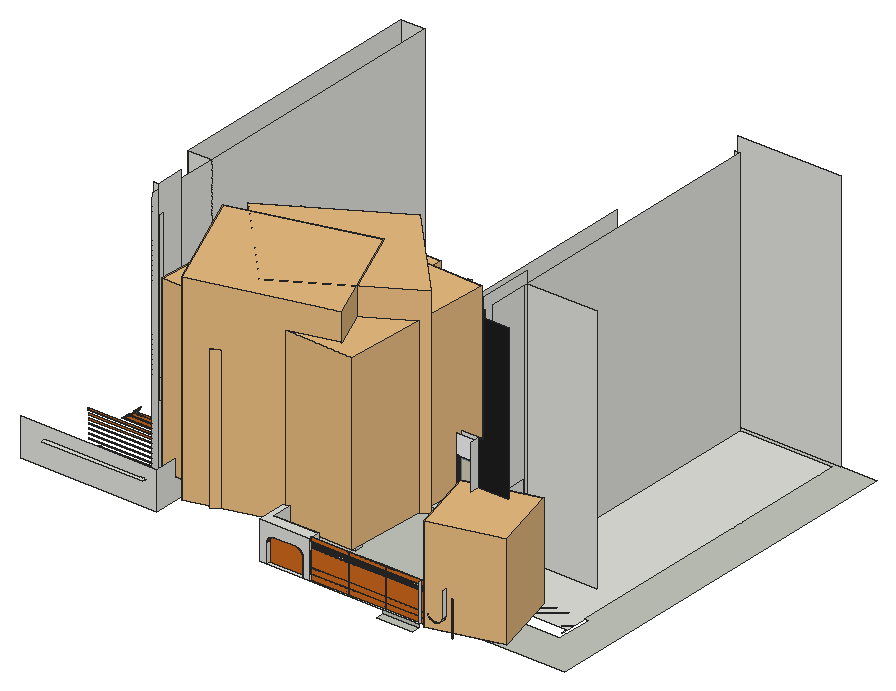
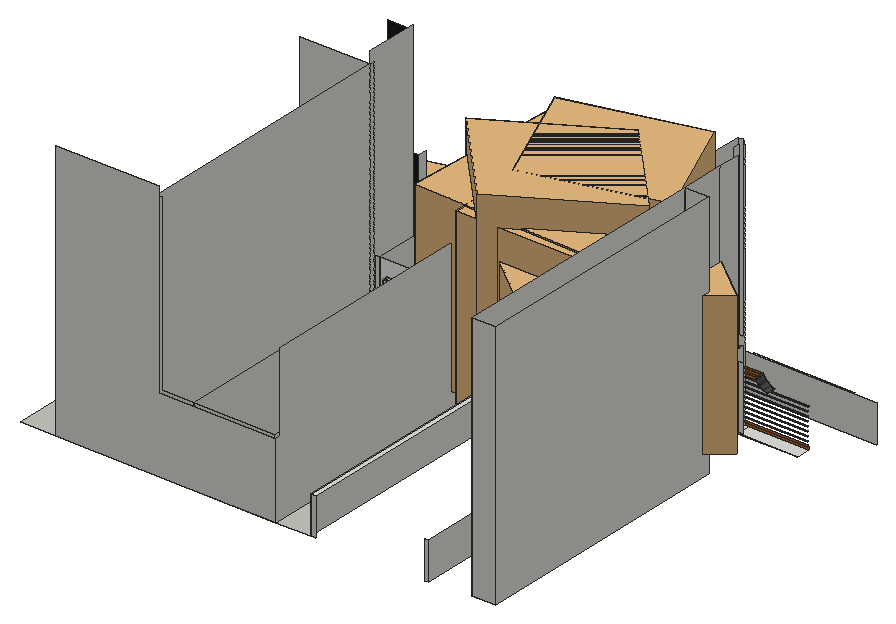
# SketchUp Ruby script. Lengths in inches.
U = 1.inch
M = Sketchup.active_model
def pt(a) = Geom::Point3d.new(a.map { |v| v * U })
def face(e, loops, mat)
  f = e.add_face(loops[0].map { |a| pt(a) })
  loops[1..].each { |l| e.add_face(l.map { |a| pt(a) }).erase! }
  f.material = f.back_material = mat if mat
  f
end
# faces: each face lists its corners as indices into pts; further lists are holes
def faces(e, pts, list, mat = nil) = list.each { |f| face(e, (f[0].is_a?(Array) ? f : [f]).map { |l| l.map { |i| pts[i] } }, mat) }
# xy, xz, yz: faces in a plane at the given z, y or x. An outline is a flat list of corners, or four numbers for a rectangle; further outlines are holes
def ring(l) = l.size == 4 ? [[l[0], l[1]], [l[2], l[1]], [l[2], l[3]], [l[0], l[3]]] : l.each_slice(2).to_a
def flat(e, list, mat, &to3) = list.each { |f| face(e, (f[0].is_a?(Array) ? f : [f]).map { |l| ring(l).map { |u, v| to3.(u, v) } }, mat) }
def xy(e, z, list, mat = nil) = flat(e, list, mat) { |x, y| [x, y, z] }
def xz(e, y, list, mat = nil) = flat(e, list, mat) { |x, z| [x, y, z] }
def yz(e, x, list, mat = nil) = flat(e, list, mat) { |y, z| [x, y, z] }
def lines(e, pts, list) = list.each { |a, b| e.add_line(pt(pts[a]), pt(pts[b])) }
# prism: a flat outline (further loops are holes) pulled along v
def prism(e, loops, v, mat = nil)
  f = face(e, loops, mat); d = Geom::Vector3d.new(v.map { |x| x * U })
  f.pushpull(f.normal.samedirection?(d) ? d.length : -d.length)
end
def box(e, o, s, mat = nil) = prism(e, [[o, [o[0] + s[0], o[1], o[2]], [o[0] + s[0], o[1] + s[1], o[2]], [o[0], o[1] + s[1], o[2]]]], [0, 0, s[2]], mat)
def at(x, y, z, deg = 0) = Geom::Transformation.translation(pt([x, y, z])) * Geom::Transformation.rotation(ORIGIN, Z_AXIS, deg.degrees)
def axes(o, x, y, z) = Geom::Transformation.new([*x, 0, *y, 0, *z, 0, *pt(o).to_a, 1])
def part(name) = M.definitions.add(name)
# library, detail: a bought-in or finely detailed component or shape, given as its bounding box
def library(name, o, s) = part(name).tap { |d| box(d.entities, o, s) }
def detail(e, o, s) = box(e.add_group.entities, o, s)
def put(e, d, t, mat = nil) = e.add_instance(d, t).tap { |i| i.material = mat if mat }
def group(e, t, mat = nil) = e.add_group.tap { |g| g.transformation = t; g.material = mat if mat }.entities
root = M.entities
M.materials.add("[0041_Chocolate]").color = [210, 105, 30]
M.materials.add("[0129_WhiteSmoke]").color = [245, 245, 245]
M.materials.add("[Color M06]").color = [84, 84, 84]
M.materials.add("[Color M08]").color = [30, 30, 30]
M.materials.add("[Pavers with Grass Herringbone]").color = [197, 201, 190]
M.materials.add("[Translucent Glass Safety]").color = [204, 235, 244]
M.materials["[Translucent Glass Safety]"].alpha = 0.5
M.materials.add("[Wood Veneer 01]").color = [120, 70, 37]
M.materials.add("[Wood Veneer 01]2").color = [94, 55, 29]
c1 = library("Group\#287",[-33.32,-34.9375,32.67],[162.87,159.66,128.34])
c2 = library("Group\#288",[-10.45,-6.67,0],[121.7,116.61,164.95])
c3 = library("Group\#286",[-10.45,-6.67,0],[121.7,116.61,164.95])
c4 = library("Group\#284",[-10.45,-6.67,0],[121.7,116.61,164.95])
c5 = library("Group\#283",[-33.32,-34.9375,32.67],[162.87,159.66,128.34])
c6 = library("Group\#285",[-33.32,-34.9375,81.35],[162.87,159.66,79.66])
c7 = library("Group\#282",[-33.32,-34.9375,77.91],[162.87,159.66,83.1])
c8 = part("Palem Elek")
put(c8.entities,c1,axes([92.2,20.3,-29.73],[0.70711,0.70711,0],[-0.70711,0.70711,0],[0,0,0.91208]))
put(c8.entities,c2,axes([60.27,20.78,0],[1,0,0],[0,1,0],[0,0,0.85762]))
put(c8.entities,c3,at(25.45,60.83,0,-53.5))
put(c8.entities,c4,at(84.4375,135.48,0,-161.4))
put(c8.entities,c5,axes([38.54,105.7,-36.19],[-0.04013,-0.99919,0],[0.99919,-0.04013,0],[0,0,1.11001]))
put(c8.entities,c6,axes([57.15,96.51,-54.45],[-0.02003,-0.49872,0.02965],[0.4996,-0.02007,0],[0.00123,0.03065,0.51628]))
put(c8.entities,c7,axes([74.94,50.39,-54.06],[0.40095,0.29715,0.03075],[-0.29654,0.38966,0.10114],[0.04012,-0.11026,0.54246]))
c9 = part("palem elek\#1")
put(c9.entities,c8,at(-81.14,-74.56,-0.83))
c10 = part("Coqueiro")
put(c10.entities,c9,axes([83.17,89.39,9.5625],[0,1.1016,0],[-1.377,0,0],[0,0,1.39284]))
c11 = part("Slatted screen panel")
xy(c11.entities,0,[[0,0,255.91,1.97]],"[Wood Veneer 01]2")
xy(c11.entities,16.54,[[0,1.18,255.91,1.97]],"[Wood Veneer 01]2")
xy(c11.entities,16.93,[[0,0,255.91,1.18]],"[Wood Veneer 01]2")
xy(c11.entities,17.78,[[0,0,255.91,1.18]],"[Wood Veneer 01]2")
xy(c11.entities,34.45,[[0,0,255.91,1.18]],"[Wood Veneer 01]2")
xy(c11.entities,35.07,[[0,0,255.91,1.18]],"[Wood Veneer 01]2")
xy(c11.entities,89.37,[[0,0,255.91,1.97]],"[Wood Veneer 01]2")
xy(c11.entities,92.91,[[0,0,255.91,1.97]],"[Wood Veneer 01]2")
xy(c11.entities,94.49,[[0,0,255.91,1.97]],"[Wood Veneer 01]2")
xy(c11.entities,97.64,[[0,0,255.91,1.97]],"[Wood Veneer 01]2")
xy(c11.entities,99.21,[[0,0,255.91,1.97]],"[Wood Veneer 01]2")
xy(c11.entities,102.36,[[0,0,255.91,1.97]],"[Wood Veneer 01]2")
xy(c11.entities,103.9375,[[0,0,255.91,1.97]],"[Wood Veneer 01]2")
xy(c11.entities,107.48,[[0,0,255.91,1.97]],"[Wood Veneer 01]2")
xy(c11.entities,119.29,[[0,0,255.91,1.97]],"[Wood Veneer 01]2")
xz(c11.entities,0,[[0,0,255.91,16.93],[0,17.78,255.91,34.45],[0,35.07,255.91,89.37],[0,92.91,255.91,94.49],[0,97.64,255.91,99.21],
  [0,102.36,255.91,103.9375],[0,107.48,255.91,119.29]],"[0041_Chocolate]")
xz(c11.entities,1.18,[[0,16.54,255.91,16.93],[0,16.93,255.91,17.78],[0,34.45,255.91,35.07]],"[Wood Veneer 01]2")
xz(c11.entities,1.97,[[0,0,255.91,1.57],[0,1.57,255.91,5.51],[0,5.51,255.91,7.09],[0,7.09,255.91,11.8125],[0,11.8125,255.91,16.54],
  [0,16.54,255.91,19.69],[0,19.69,255.91,89.37],[0,92.91,255.91,94.49],[0,97.64,255.91,99.21],[0,102.36,255.91,103.9375],
  [0,107.48,255.91,109.84],[0,109.84,255.91,119.29]],"[Wood Veneer 01]2")
yz(c11.entities,0,[[0,0,1.97,1.57],[0,1.57,1.97,5.51],[0,5.51,1.97,7.09],[0,7.09,1.97,11.8125],[0,11.8125,0,16.93,1.18,16.93,1.18,16.54,1.97,16.54,1.97,11.8125],
  [1.18,16.54,1.97,19.69],[0,17.78,0,34.45,1.18,34.45,1.18,35.07,0,35.07,0,89.37,1.97,89.37,1.97,19.69,1.18,19.69,1.18,17.78],[0,92.91,1.97,94.49],[0,97.64,1.97,99.21],[0,102.36,1.97,103.9375],
  [0,107.48,1.97,109.84],[0,109.84,1.97,119.29]],"[Wood Veneer 01]2")
yz(c11.entities,255.91,[[0,0,1.97,1.57],[0,1.57,1.97,5.51],[0,5.51,1.97,7.09],[0,7.09,1.97,11.8125],[0,11.8125,1.97,11.8125,1.97,16.54,1.18,16.54,1.18,16.93,0,16.93],
  [1.18,16.54,1.97,19.69],[0,17.78,1.18,17.78,1.18,19.69,1.97,19.69,1.97,89.37,0,89.37,0,35.07,1.18,35.07,1.18,34.45,0,34.45],[0,92.91,1.97,94.49],[0,97.64,1.97,99.21],[0,102.36,1.97,103.9375],
  [0,107.48,1.97,109.84],[0,109.84,1.97,119.29]],"[Wood Veneer 01]2")
p = [[255.91,1.97,103.9375],[255.91,1.97,107.48],[0,1.97,107.48],[0,1.97,103.9375],[0,1.97,92.91],[0,1.97,89.37],
  [255.91,1.97,99.21],[255.91,1.97,102.36],[255.91,1.97,89.37],[255.91,1.97,92.91],[0,1.97,97.64],[0,1.97,94.49],
  [0,1.97,102.36],[0,1.97,99.21],[255.91,1.97,94.49],[255.91,1.97,97.64],[240.94,0,5.51],[240.94,1.97,5.51]]
lines(c11.entities,p,[[0,1],[2,3],[4,5],[6,7],[8,9],[10,11],[12,13],[14,15],[16,17]])
c12 = part("Group\#3")
g1 = group(c12.entities,at(0,0,0))
xy(g1,0,[[0,0,6,48]],"[Wood Veneer 01]")
xy(g1,4,[[0,4,1.8125,44],[1.8125,4,6,44]])
xy(g1,80,[[0,4,1.8125,44],[1.8125,4,6,44]])
xy(g1,84,[[0,0,6,48]],"[Wood Veneer 01]")
xz(g1,0,[[0,0,6,84]],"[Wood Veneer 01]")
xz(g1,4,[[0,4,1.8125,80],[1.8125,4,6,80]])
xz(g1,44,[[0,4,1.8125,80],[1.8125,4,6,80]])
xz(g1,48,[[0,0,6,84]],"[Wood Veneer 01]")
yz(g1,0,[[[0,0,48,84],[4,4,44,80]]],"[Wood Veneer 01]")
yz(g1,1.8125,[[4,4,44,80]],"[Translucent Glass Safety]")
yz(g1,6,[[[0,0,48,84],[4,4,44,80]]],"[Wood Veneer 01]")
g2 = group(c12.entities,at(0,48,0))
xy(g2,0,[[0,0,6,48]],"[Wood Veneer 01]")
xy(g2,4,[[0,4,1.8125,44],[1.8125,4,6,44]])
xy(g2,80,[[0,4,1.8125,44],[1.8125,4,6,44]])
xy(g2,84,[[0,0,6,48]],"[Wood Veneer 01]")
xz(g2,0,[[0,0,6,84]],"[Wood Veneer 01]")
xz(g2,4,[[0,4,1.8125,80],[1.8125,4,6,80]])
xz(g2,44,[[0,4,1.8125,80],[1.8125,4,6,80]])
xz(g2,48,[[0,0,6,84]],"[Wood Veneer 01]")
yz(g2,0,[[[0,0,48,84],[4,4,44,80]]],"[Wood Veneer 01]")
yz(g2,1.8125,[[4,4,44,80]],"[Translucent Glass Safety]")
yz(g2,6,[[[0,0,48,84],[4,4,44,80]]],"[Wood Veneer 01]")
c13 = library("元件\#5",[-4.39,0,0],[5.37,35.83,90.55])
c14 = library("Palm tree",[-4.09,-4.52,0],[193.52,193.51,258.93])
c15 = part("Palm+Tree")
put(c15.entities,c14,at(25.51,-21.81,0,15))
xy(root,0.73,[[1432.9,185.9375,1489.92,198.625]],"[Pavers with Grass Herringbone]")
xy(root,6.125,[[1247.55,198.625,1304.42,204.875],[1315.36,198.625,1490.16,217.125],[897.21,280.47,992.73,280.47,992.73,292.45,991.85,292.45,991.85,302.0625,897.21,302.0625],[992.73,280.47,998.64,292.45],[991.85,292.45,992.73,302.46],
  [992.73,292.45,999.52,302.46],[1486.5,292.45,1498.09,292.45,1498.09,305.58,1547.21,305.58,1547.21,292.45,1547.71,292.45,1547.71,302.0625,1642.35,302.0625,1642.35,292.45,1643.23,292.45,1643.23,830.91,1306.63,830.91,1306.63,448.51,1436.71,448.51,1436.71,406.38,1495.03,406.38,1495.03,397.86,1486.5,397.86],[1486.5,292.45,1498.09,305.58],[1299.4,294.33,1312.4,305.58],[897.21,302.0625,991.85,302.46],
  [992.73,302.46,999.52,305.58],[992.73,305.58,999.52,336.27],[1486.5,305.58,1498.09,312.8125],[1547.71,305.58,1547.71,312.8125,1496.21,312.8125,1496.21,336.27,1643.23,336.27,1643.23,305.58],[1498.09,305.58,1507.74,312.8125],
  [1486.5,312.8125,1486.5,397.86,1495.03,397.86,1495.03,321.34,1496.21,321.34,1496.21,312.8125],[1495.03,321.34,1496.21,397.86],[1496.21,337.5625,1643.23,337.5625,1643.23,406.38,1495.03,406.38,1495.03,399.07,1496.21,399.07],[1495.03,397.86,1496.21,399.07],[955.73,406.38,992.73,830.91],
  [1436.71,406.38,1495.03,830.91],[1306.63,448.51,1436.71,830.91]])
xy(root,6.125,[[[1244.07,217.125,1707,217.125,1707,838.14,1299.4,838.14,1299.4,439.98,1417.88,439.98,1417.88,397.86,1427.92,397.86,1427.92,405.05,1475.11,405.05,1475.11,397.86,1495.03,397.86,1495.03,406.38,1436.71,406.38,1436.71,448.51,1306.63,448.51,1306.63,830.91,1643.23,830.91,1643.23,336.27,1650.02,336.27,1650.02,292.45,1649.14,292.45,1649.14,280.47,1547.71,280.47,1547.71,292.45,1547.21,292.45,1547.21,305.58,1498.09,305.58,1498.09,292.45,1486.5,292.45,1486.5,397.86,1475.11,397.86,1475.11,405.05,1427.92,405.05,1427.92,397.86,1417.88,397.86,1417.88,439.98,1299.4,439.98,1299.4,838.14,1244.07,838.14],[1299.4,294.33,1312.4,305.58]]],"[Pavers with Grass Herringbone]")
xy(root,40.13,[[1335.37,439.98,1383,448.51]])
xy(root,48,[[1258.48,198.625,1292.93,204.875]])
xy(root,55.1875,[[888.5,198.625,888.5,203.875,890.125,203.875,890.125,204.875,890.875,204.875,890.875,203.875,894.125,203.875,894.125,204.875,894.875,204.875,894.875,203.875,898.125,203.875,898.125,204.875,898.875,204.875,898.875,203.875,902.125,203.875,902.125,204.875,902.875,204.875,902.875,203.875,906.125,203.875,906.125,204.875,906.875,204.875,906.875,203.875,910.125,203.875,910.125,204.875,910.875,204.875,910.875,203.875,914.125,203.875,914.125,204.875,914.875,204.875,914.875,203.875,918.125,203.875,918.125,204.875,918.875,204.875,918.875,203.875,922.125,203.875,922.125,204.875,922.875,204.875,922.875,203.875,926.125,203.875,926.125,204.875,926.875,204.875,926.875,203.875,930.125,203.875,930.125,204.875,930.875,204.875,930.875,203.875,934.125,203.875,934.125,204.875,934.875,204.875,934.875,203.875,938.125,203.875,938.125,204.875,938.875,204.875,938.875,203.875,942.125,203.875,942.125,204.875,942.875,204.875,942.875,203.875,946.125,203.875,946.125,204.875,946.875,204.875,946.875,203.875,950.125,203.875,950.125,204.875,950.875,204.875,950.875,203.875,954.125,203.875,954.125,204.875,954.875,204.875,954.875,203.875,958.125,203.875,958.125,204.875,958.875,204.875,958.875,203.875,962.125,203.875,962.125,204.875,962.875,204.875,962.875,203.875,966.125,203.875,966.125,204.875,966.875,204.875,966.875,203.875,970.125,203.875,970.125,204.875,970.875,204.875,970.875,203.875,974.125,203.875,974.125,204.875,974.875,204.875,974.875,203.875,978.125,203.875,978.125,204.875,978.875,204.875,978.875,203.875,982.125,203.875,982.125,204.875,982.875,204.875,982.875,203.875,986.125,203.875,986.125,204.875,986.875,204.875,986.875,203.875,990.125,203.875,990.125,204.875,990.875,204.875,990.875,203.875,994.125,203.875,994.125,204.875,994.875,204.875,994.875,203.875,998.125,203.875,998.125,204.875,998.875,204.875,998.875,203.875,1002.125,203.875,1002.125,204.875,1002.875,204.875,1002.875,203.875,1006.125,203.875,1006.125,204.875,1006.875,204.875,1006.875,203.875,1010.125,203.875,1010.125,204.875,1010.875,204.875,1010.875,203.875,1014.125,203.875,1014.125,204.875,1014.875,204.875,1014.875,203.875,1018.125,203.875,1018.125,204.875,1018.875,204.875,1018.875,203.875,1022.125,203.875,1022.125,204.875,1022.875,204.875,1022.875,203.875,1026.125,203.875,1026.125,204.875,1026.875,204.875,1026.875,203.875,1030.125,203.875,1030.125,204.875,1030.875,204.875,1030.875,203.875,1034.125,203.875,1034.125,204.875,1034.875,204.875,1034.875,203.875,1038.125,203.875,1038.125,204.875,1038.875,204.875,1038.875,203.875,1042.125,203.875,1042.125,204.875,1042.875,204.875,1042.875,203.875,1046.125,203.875,1046.125,204.875,1046.875,204.875,1046.875,203.875,1050.125,203.875,1050.125,198.625]])
xy(root,66.125,[[1235.9,198.625,1315.36,198.625,1315.36,217.125,1244.07,217.125,1244.07,838.14,1235.9,838.14]])
xy(root,67.58,[[897.21,280.47,998.64,281.47]],"[0041_Chocolate]")
xy(root,69.6875,[[897.21,280.47,998.64,281.47]],"[0041_Chocolate]")
xy(root,74.64,[[951.36,280.47,998.64,281.47]],"[0041_Chocolate]")
xy(root,76.75,[[956.45,280.47,998.64,281.47]],"[0041_Chocolate]")
xy(root,81.7,[[963.29,280.47,998.64,281.47]],"[0041_Chocolate]")
xy(root,83.8125,[[964.97,280.47,998.64,281.47]],"[0041_Chocolate]")
xy(root,88.77,[[968.5,280.47,998.64,281.47]],"[0041_Chocolate]")
xz(root,198.625,[[1235.9,6.125,1247.55,6.125,1247.55,37.07,1247.64,38.5,1247.92,39.9,1248.38,41.25,1249.01,42.53,1249.81,43.72,1250.75,44.8,1251.82,45.74,1253.01,46.54,1254.3,47.17,1255.65,47.63,1257.05,47.91,1258.48,48,1292.93,48,1294.43,47.9,1295.9,47.61,1297.33,47.125,1298.68,46.46,1299.93,45.625,1301.06,44.63,1302.05,43.5,1302.88,42.25,1303.55,40.9,1304.03,39.48,1304.32,38.01,1304.42,36.51,1304.42,6.125,1315.36,6.125,1315.36,66.125,1235.9,66.125]])
xz(root,198.625,[[1432.9,0.73,1489.92,6.125]],"[Pavers with Grass Herringbone]")
xz(root,204.875,[[1537.375,0,1539,55.1875]])
xz(root,204.875,[[1247.55,6.125,1304.42,6.125,1304.42,36.51,1304.32,38.01,1304.03,39.48,1303.55,40.9,1302.88,42.25,1302.05,43.5,1301.06,44.63,1299.93,45.625,1298.68,46.46,1297.33,47.125,1295.9,47.61,1294.43,47.9,1292.93,48,1258.48,48,1257.05,47.91,1255.65,47.63,1254.3,47.17,1253.01,46.54,1251.82,45.74,1250.75,44.8,1249.81,43.72,1249.01,42.53,1248.38,41.25,1247.92,39.9,1247.64,38.5,1247.55,37.07],[1515.44,16.91,1518.24,17.23,1520.9,18.17,1523.27,19.69,1525.24,21.71,1526.71,24.11,1527.6,26.79,1527.6,66.125,1503.29,66.125,1503.29,26.79,1504.17,24.11,1505.64,21.71,1507.61,19.69,1509.99,18.17,1512.64,17.23]],"[0041_Chocolate]")
xz(root,217.125,[[839.66,6.125,1056.5,66.125],[1244.07,6.125,1315.36,66.125]])
xz(root,280.47,[[897.21,6.125,998.64,11.08],[956.45,76.75,998.64,76.75,998.64,81.7,963.29,81.7,957.28,77.09],[964.97,83.8125,998.64,83.8125,998.64,88.77,968.5,88.77,968.18,88]],"[0041_Chocolate]")
xz(root,281.47,[[897.21,11.08,998.64,13.1875],[897.21,18.14,998.64,20.25],[897.21,25.2,998.64,27.3125],[897.21,32.27,998.64,34.375],[897.21,39.33,998.64,41.4375],
  [897.21,46.39,998.64,48.5],[897.21,53.45,998.64,55.5625],[897.21,60.52,998.64,62.625],[897.21,67.58,998.64,69.6875],[951.36,74.64,998.64,74.64,998.64,76.75,956.45,76.75],
  [963.29,81.7,998.64,81.7,998.64,83.8125,964.97,83.8125,963.45,81.83],[968.5,88.77,998.64,88.77,998.64,90.875,969.37,90.875]],"[0041_Chocolate]")
xz(root,292.45,[[991.85,6.125,992.73,126.125],[992.73,6.125,998.64,126.125],[998.64,6.125,999.52,6.125,999.52,421.25,992.73,421.25,992.73,141.26,998.64,141.26]])
xz(root,292.45,[[1486.5,6.125,1498.09,132.47]],"[0129_WhiteSmoke]")
xz(root,294.33,[[1299.4,6.125,1312.4,128.75]],"[0129_WhiteSmoke]")
xz(root,302.46,[[984.18,6.125,991.85,8.32],[991.85,6.125,992.73,8.32],[992.73,6.125,999.52,8.32],[1547.21,6.125,1547.71,8.32],[984.18,8.32,991.85,109.9375],
  [991.85,8.32,992.73,109.9375],[1547.21,8.32,1547.71,95.62]])
xz(root,305.58,[[1299.4,6.125,1312.4,128.75]])
xz(root,305.58,[[1498.09,6.125,1547.21,6.125,1547.21,126.125,1547.71,126.125,1547.71,402.64,1507.74,402.64,1507.74,226.8,1498.09,226.8]],"[Color M08]")
xz(root,312.8125,[[1496.21,6.125,1498.09,126.125],[1498.09,6.125,1507.74,126.125]])
xz(root,321.34,[[1495.03,6.125,1496.21,402.64]])
xz(root,397.86,[[1486.5,6.125,1496.21,126.125]])
xz(root,397.86,[[1417.88,6.125,1427.92,6.125,1427.92,101.1875,1475.11,101.1875,1475.11,6.125,1486.5,6.125,1486.5,126.125,1417.88,126.125]],"[0129_WhiteSmoke]")
xz(root,399.07,[[1495.03,6.125,1496.21,402.64]])
xz(root,405.05,[[1427.92,6.125,1475.11,101.1875]])
xz(root,406.38,[[955.73,6.125,992.73,402.64],[1495.03,6.125,1606.23,402.64]])
xz(root,439.98,[[[1299.4,6.125,1417.88,126.125],[1335.37,40.13,1383,95.51]]],"[0129_WhiteSmoke]")
xz(root,448.51,[[1306.63,6.125,1315.15,126.125],[[1315.15,6.125,1436.71,126.125],[1335.37,40.13,1383,95.51]]])
xz(root,830.91,[[955.73,6.125,992.73,402.64],[1306.63,6.125,1436.71,126.125],[1436.71,6.125,1436.71,126.125,1486.5,126.125,1486.5,402.64,1495.03,402.64,1495.03,6.125]])
xz(root,838.14,[[1056.5,6.125,1063.02,66.125],[1235.9,6.125,1244.07,66.125],[1299.4,6.125,1299.4,126.125,1486.5,126.125,1486.5,421.25,1650.02,421.25,1650.02,6.125]])
yz(root,955.73,[[406.38,6.125,830.91,402.64]])
yz(root,991.85,[[292.45,6.125,302.46,126.125]])
yz(root,992.73,[[302.46,6.125,337.5625,402.64],[337.5625,6.125,406.38,402.64],[406.38,6.125,830.91,402.64]])
yz(root,998.64,[[280.47,6.125,292.45,6.125,292.45,141.26,302.46,141.26,302.46,411.82,281.47,411.82,281.47,405.64,280.47,405.64,280.47,400.6875,281.47,400.6875,281.47,398.77,280.47,398.77,280.47,393.8125,281.47,393.8125,281.47,391.89,280.47,391.89,280.47,386.9375,281.47,386.9375,281.47,385.02,280.47,385.02,280.47,380.0625,281.47,380.0625,281.47,378.14,280.47,378.14,280.47,373.1875,281.47,373.1875,281.47,371.27,280.47,371.27,280.47,366.3125,281.47,366.3125,281.47,364.2,280.47,364.2,280.47,359.25,281.47,359.25,281.47,357.14,280.47,357.14,280.47,352.1875,281.47,352.1875,281.47,350.08,280.47,350.08,280.47,345.125,281.47,345.125,281.47,343.02,280.47,343.02,280.47,338.0625,281.47,338.0625,281.47,335.95,280.47,335.95,280.47,331,281.47,331,281.47,328.89,280.47,328.89,280.47,323.9375,281.47,323.9375,281.47,321.83,280.47,321.83,280.47,316.875,281.47,316.875,281.47,314.77,280.47,314.77,280.47,309.8125,281.47,309.8125,281.47,307.7,280.47,307.7,280.47,302.75,281.47,302.75,281.47,300.64,280.47,300.64,280.47,295.6875,281.47,295.6875,281.47,293.58,280.47,293.58,280.47,288.625,281.47,288.625,281.47,286.52,280.47,286.52,280.47,281.5625,281.47,281.5625,281.47,279.45,280.47,279.45,280.47,274.5,281.47,274.5,281.47,272.39,280.47,272.39,280.47,267.4375,281.47,267.4375,281.47,265.33,280.47,265.33,280.47,260.375,281.47,260.375,281.47,258.27,280.47,258.27,280.47,253.3125,281.47,253.3125,281.47,251.2,280.47,251.2,280.47,246.25,281.47,246.25,281.47,244.14,280.47,244.14,280.47,239.1875,281.47,239.1875,281.47,237.08,280.47,237.08,280.47,232.125,281.47,232.125,281.47,230.02,280.47,230.02,280.47,225.0625,281.47,225.0625,281.47,222.95,280.47,222.95,280.47,218,281.47,218,281.47,215.89,280.47,215.89,280.47,210.9375,281.47,210.9375,281.47,208.83,280.47,208.83,280.47,203.875,281.47,203.875,281.47,201.77,280.47,201.77,280.47,196.8125,281.47,196.8125,281.47,194.7,280.47,194.7,280.47,189.75,281.47,189.75,281.47,187.64,280.47,187.64,280.47,182.6875,281.47,182.6875,281.47,180.58,280.47,180.58,280.47,175.625,281.47,175.625,281.47,173.52,280.47,173.52,280.47,168.5625,281.47,168.5625,281.47,166.45,280.47,166.45,280.47,161.5,281.47,161.5,281.47,159.39,280.47,159.39,280.47,154.4375,281.47,154.4375,281.47,152.33,280.47,152.33,280.47,147.375,281.47,147.375,281.47,145.27,280.47,145.27,280.47,140.3125,281.47,140.3125,281.47,138.2,280.47,138.2,280.47,133.25,281.47,133.25,281.47,131.14,280.47,131.14,280.47,126.1875,281.47,126.1875,281.47,124.08,280.47,124.08,280.47,119.125,281.47,119.125,281.47,117.02,280.47,117.02,280.47,112.0625,281.47,112.0625,281.47,109.95,280.47,109.95,280.47,105,281.47,105,281.47,102.89,280.47,102.89,280.47,97.9375,281.47,97.9375,281.47,95.83,280.47,95.83,280.47,90.875,281.47,90.875,281.47,88.77,280.47,88.77,280.47,83.8125,281.47,83.8125,281.47,81.7,280.47,81.7,280.47,76.75,281.47,76.75,281.47,74.64,280.47,74.64,280.47,69.6875,281.47,69.6875,281.47,67.58,280.47,67.58,280.47,62.625,281.47,62.625,281.47,60.52,280.47,60.52,280.47,55.5625,281.47,55.5625,281.47,53.45,280.47,53.45,280.47,48.5,281.47,48.5,281.47,46.39,280.47,46.39,280.47,41.4375,281.47,41.4375,281.47,39.33,280.47,39.33,280.47,34.375,281.47,34.375,281.47,32.27,280.47,32.27,280.47,27.3125,281.47,27.3125,281.47,25.2,280.47,25.2,280.47,20.25,281.47,20.25,281.47,18.14,280.47,18.14,280.47,13.1875,281.47,13.1875,281.47,11.08,280.47,11.08]])
yz(root,999.52,[[292.45,6.125,336.27,6.125,336.27,421.25,292.45,421.25,292.45,376.875,302.46,376.875,302.46,109.9375,299.11,109.9375,295.02,110.21,292.45,110.72]])
yz(root,1056.5,[[217.125,6.125,838.14,66.125]])
yz(root,1244.07,[[217.125,6.125,838.14,66.125]])
yz(root,1247.55,[[198.625,6.125,204.875,37.07]])
yz(root,1299.4,[[294.33,6.125,294.33,128.75,298.39,128.75,298.39,126.125,305.58,126.125,305.58,6.125],[439.98,6.125,439.98,252.47,830.91,252.47,830.91,126.125,838.14,126.125,838.14,6.125]])
yz(root,1304.42,[[198.625,6.125,204.875,36.51]])
yz(root,1306.63,[[448.51,6.125,830.91,126.125]])
yz(root,1312.4,[[294.33,6.125,305.58,128.75]])
yz(root,1315.36,[[198.625,6.125,217.125,66.125]])
yz(root,1335.37,[[439.98,40.13,448.51,95.51]])
yz(root,1383,[[439.98,40.13,448.51,95.51]])
yz(root,1417.88,[[397.86,6.125,439.98,126.125]])
yz(root,1427.92,[[397.86,6.125,405.05,101.1875]])
yz(root,1436.71,[[406.38,6.125,448.51,126.125],[448.51,6.125,830.91,126.125]])
yz(root,1475.11,[[397.86,6.125,405.05,101.1875]])
yz(root,1486.5,[[292.45,6.125,292.45,132.47,305.58,132.47,305.58,126.125,397.86,126.125,397.86,6.125]])
yz(root,1490.16,[[198.625,6.125,217.125,66.125]])
yz(root,1495.03,[[321.34,6.125,321.34,421.25,406.38,421.25,406.38,402.64,399.07,402.64,399.07,6.125],[399.07,6.125,406.38,402.64],[406.38,6.125,830.91,402.64]])
yz(root,1496.21,[[312.8125,6.125,321.34,126.125],[321.34,6.125,336.27,126.125],[336.27,6.125,337.5625,126.125],[337.5625,6.125,397.86,126.125],[397.86,6.125,399.07,6.125,399.07,402.64,337.5625,402.64,337.5625,126.125,397.86,126.125]])
yz(root,1498.09,[[292.45,6.125,305.58,226.8]])
yz(root,1503.29,[[198.625,26.79,204.875,66.125]])
yz(root,1527.6,[[198.625,26.79,204.875,66.125]])
yz(root,1539,[[203.875,0,204.875,55.1875]])
yz(root,1547.21,[[302.46,6.125,305.58,8.32],[302.46,8.32,305.58,95.62]])
p = [[1515.44,204.875,16.91],[1512.64,204.875,17.23],[1512.64,198.625,17.23],[1515.44,198.625,16.91],[1518.24,204.875,17.23],[1518.24,198.625,17.23],
  [1509.99,204.875,18.17],[1509.99,198.625,18.17],[1520.9,204.875,18.17],[1520.9,198.625,18.17],[1507.61,204.875,19.69],[1507.61,198.625,19.69],
  [1523.27,204.875,19.69],[1523.27,198.625,19.69],[1505.64,204.875,21.71],[1505.64,198.625,21.71],[1525.24,204.875,21.71],[1525.24,198.625,21.71],
  [1504.17,204.875,24.11],[1504.17,198.625,24.11],[1526.71,204.875,24.11],[1526.71,198.625,24.11],[1503.29,204.875,26.79],[1503.29,198.625,26.79],
  [1527.6,204.875,26.79],[1527.6,198.625,26.79],[1304.32,204.875,38.01],[1304.42,204.875,36.51],[1304.42,198.625,36.51],[1304.32,198.625,38.01],
  [1247.55,204.875,37.07],[1247.64,204.875,38.5],[1247.64,198.625,38.5],[1247.55,198.625,37.07],[1304.03,204.875,39.48],[1304.03,198.625,39.48],
  [1247.92,204.875,39.9],[1247.92,198.625,39.9],[1303.55,204.875,40.9],[1303.55,198.625,40.9],[1248.38,204.875,41.25],[1248.38,198.625,41.25],
  [1302.88,204.875,42.25],[1302.88,198.625,42.25],[1249.01,204.875,42.53],[1249.01,198.625,42.53],[1302.05,204.875,43.5],[1302.05,198.625,43.5],
  [1249.81,204.875,43.72],[1249.81,198.625,43.72],[1301.06,204.875,44.63],[1301.06,198.625,44.63],[1250.75,204.875,44.8],[1250.75,198.625,44.8],
  [1299.93,204.875,45.625],[1299.93,198.625,45.625],[1251.82,204.875,45.74],[1251.82,198.625,45.74],[1298.68,204.875,46.46],[1298.68,198.625,46.46],
  [1253.01,204.875,46.54],[1253.01,198.625,46.54],[1254.3,204.875,47.17],[1254.3,198.625,47.17],[1297.33,204.875,47.125],[1297.33,198.625,47.125],
  [1295.9,204.875,47.61],[1295.9,198.625,47.61],[1255.65,204.875,47.63],[1255.65,198.625,47.63],[1257.05,204.875,47.91],[1257.05,198.625,47.91],
  [1294.43,204.875,47.9],[1294.43,198.625,47.9],[1258.48,204.875,48],[1258.48,198.625,48],[1292.93,204.875,48],[1292.93,198.625,48],
  [950.09,295.65,74.12],[950.09,280.47,74.12],[951.36,280.47,74.64],[951.36,281.47,74.64],[951.36,295.65,74.64],[956.45,281.47,76.75],
  [956.45,295.65,76.75],[956.45,280.47,76.75],[957.28,280.47,77.09],[957.28,295.65,77.09],[963.29,280.47,81.7],[963.29,281.47,81.7],
  [963.29,295.65,81.7],[963.45,281.47,81.83],[963.45,295.65,81.83],[964.97,281.47,83.8125],[964.97,295.65,83.8125],[964.97,280.47,83.8125],
  [968.18,280.47,88],[968.18,295.65,88],[968.5,280.47,88.77],[968.5,281.47,88.77],[968.5,295.65,88.77],[969.37,281.47,90.875],
  [969.37,295.65,90.875]]
faces(root,p,[[0,1,2,3],[4,0,3,5],[1,6,7,2],[8,4,5,9],[6,10,11,7],[12,8,9,13],[10,14,15,11],[16,12,13,17],
  [14,18,19,15],[20,16,17,21],[18,22,23,19],[24,20,21,25],[26,27,28,29],[30,31,32,33],[34,26,29,35],[31,36,37,32],
  [38,34,35,39],[36,40,41,37],[42,38,39,43],[40,44,45,41],[46,42,43,47],[44,48,49,45],[50,46,47,51],[48,52,53,49],
  [54,50,51,55],[52,56,57,53],[58,54,55,59],[56,60,61,57],[60,62,63,61],[64,58,59,65],[66,64,65,67],[62,68,69,63],
  [68,70,71,69],[72,66,67,73],[70,74,75,71],[76,72,73,77]])
faces(root,p,[[78,79,80,81,82],[81,83,84,82],[84,83,85,86,87],[87,86,88,89,90],[89,91,92,90],[91,93,94,92],[94,93,95,96,97],[97,96,98,99,100],
  [99,101,102,100]],"[Color M06]")
put(root,c10,axes([1046.32,246.74,29.13],[1.38444,0,0],[0,1.38444,0],[0,0,1.38444]))
put(root,c11,axes([1315.46,201.88,6.125],[0.23355,0,0],[0,0.5124,0],[0,0,0.5124]),"[0041_Chocolate]")
put(root,c12,axes([1335.37,442.86,40.13],[0,-0.48,0],[0.49609,0,0],[0,0,0.65923]))
put(root,c11,axes([1375.23,201.88,6.125],[0.23355,0,0],[0,0.5124,0],[0,0,0.5124]),"[Pavers with Grass Herringbone]")
put(root,c13,axes([1427.92,398.25,6.11],[0,-1.05,0],[1.302,0,0],[0,0,1.05]))
put(root,c11,axes([1434.99,201.88,6.125],[0.23355,0,0],[0,0.5124,0],[0,0,0.5124]),"[0041_Chocolate]")
put(root,c15,axes([1485.79,212.94,6.125],[0.58344,0,0],[0,0.58344,0],[0,0,0.58344]),"[Color M06]")
